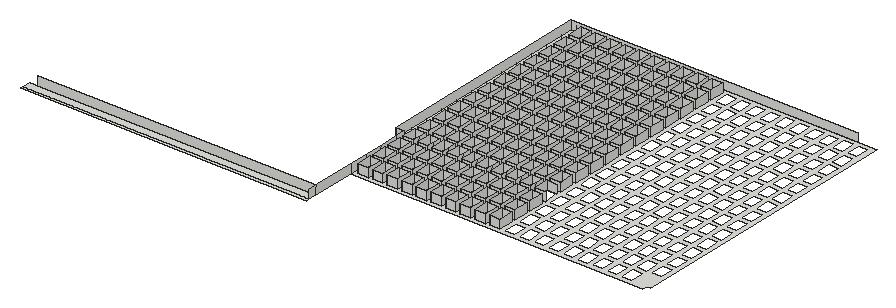
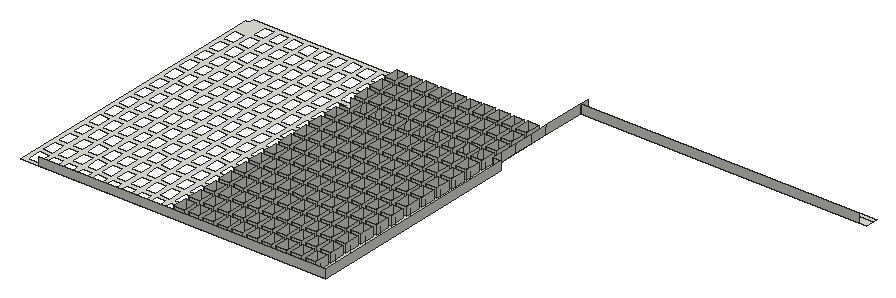
# SketchUp Ruby script. Lengths in inches.
U = 1.inch
M = Sketchup.active_model
def pt(a) = Geom::Point3d.new(a.map { |v| v * U })
def face(e, loops, mat)
  f = e.add_face(loops[0].map { |a| pt(a) })
  loops[1..].each { |l| e.add_face(l.map { |a| pt(a) }).erase! }
  f.material = f.back_material = mat if mat
  f
end
# faces: each face lists its corners as indices into pts; further lists are holes
def faces(e, pts, list, mat = nil) = list.each { |f| face(e, (f[0].is_a?(Array) ? f : [f]).map { |l| l.map { |i| pts[i] } }, mat) }
# xy, xz, yz: faces in a plane at the given z, y or x. An outline is a flat list of corners, or four numbers for a rectangle; further outlines are holes
def ring(l) = l.size == 4 ? [[l[0], l[1]], [l[2], l[1]], [l[2], l[3]], [l[0], l[3]]] : l.each_slice(2).to_a
def flat(e, list, mat, &to3) = list.each { |f| face(e, (f[0].is_a?(Array) ? f : [f]).map { |l| ring(l).map { |u, v| to3.(u, v) } }, mat) }
def xy(e, z, list, mat = nil) = flat(e, list, mat) { |x, y| [x, y, z] }
def xz(e, y, list, mat = nil) = flat(e, list, mat) { |x, z| [x, y, z] }
def yz(e, x, list, mat = nil) = flat(e, list, mat) { |y, z| [x, y, z] }
def lines(e, pts, list) = list.each { |a, b| e.add_line(pt(pts[a]), pt(pts[b])) }
# prism: a flat outline (further loops are holes) pulled along v
def prism(e, loops, v, mat = nil)
  f = face(e, loops, mat); d = Geom::Vector3d.new(v.map { |x| x * U })
  f.pushpull(f.normal.samedirection?(d) ? d.length : -d.length)
end
def box(e, o, s, mat = nil) = prism(e, [[o, [o[0] + s[0], o[1], o[2]], [o[0] + s[0], o[1] + s[1], o[2]], [o[0], o[1] + s[1], o[2]]]], [0, 0, s[2]], mat)
def at(x, y, z, deg = 0) = Geom::Transformation.translation(pt([x, y, z])) * Geom::Transformation.rotation(ORIGIN, Z_AXIS, deg.degrees)
def axes(o, x, y, z) = Geom::Transformation.new([*x, 0, *y, 0, *z, 0, *pt(o).to_a, 1])
def part(name) = M.definitions.add(name)
# library, detail: a bought-in or finely detailed component or shape, given as its bounding box
def library(name, o, s) = part(name).tap { |d| box(d.entities, o, s) }
def detail(e, o, s) = box(e.add_group.entities, o, s)
def put(e, d, t, mat = nil) = e.add_instance(d, t).tap { |i| i.material = mat if mat }
def group(e, t, mat = nil) = e.add_group.tap { |g| g.transformation = t; g.material = mat if mat }.entities
root = M.entities
xy(root,246,[[189.37,0.36,387.37,2.36],[189.37,2.36,387.37,8.36],[[387.37,38.27,387.37,84.36,381.37,84.36,381.37,236.18,592.3,236.18,592.3,41,589.58,41,589.58,38.27],[582.19,54.01,589.58,64.3],[582.19,93.05,589.58,103.33],[582.19,106.06,589.58,116.34],[582.19,223.16,589.58,233.45],[582.19,184.13,589.58,194.41],[582.19,145.09,589.58,155.38],[572.08,54.01,579.47,64.3],[572.08,93.05,579.47,103.33],[572.08,106.06,579.47,116.34],[572.08,145.09,579.47,155.38],[572.08,184.13,579.47,194.41],[572.08,223.16,579.47,233.45],[561.97,223.16,569.35,233.45],[561.97,184.13,569.35,194.41],[561.97,171.12,569.35,181.4],[561.97,145.09,569.35,155.38],[561.97,106.06,569.35,116.34],[561.97,93.05,569.35,103.33],[561.97,54.01,569.35,64.3],[390.09,223.16,397.48,233.45],[400.2,223.16,407.59,233.45],[400.2,184.13,407.59,194.41],[400.2,171.12,407.59,181.4],[400.2,145.09,407.59,155.38],[400.2,106.06,407.59,116.34],[400.2,93.05,407.59,103.33],[400.2,54.01,407.59,64.3],[410.3125,54.01,417.7,64.3],[410.3125,93.05,417.7,103.33],[410.3125,106.06,417.7,116.34],[410.3125,145.09,417.7,155.38],[410.3125,184.13,417.7,194.41],[410.3125,223.16,417.7,233.45],[420.42,223.16,427.81,233.45],[420.42,184.13,427.81,194.41],[420.42,145.09,427.81,155.38],[420.42,106.06,427.81,116.34],[420.42,93.05,427.81,103.33],[420.42,54.01,427.81,64.3],[430.53,223.16,437.92,233.45],[430.53,184.13,437.92,194.41],[430.53,145.09,437.92,155.38],[430.53,106.06,437.92,116.34],[430.53,93.05,437.92,103.33],[430.53,54.01,437.92,64.3],[440.64,54.01,448.03,64.3],[440.64,93.05,448.03,103.33],[440.64,106.06,448.03,116.34],[440.64,145.09,448.03,155.38],[440.64,184.13,448.03,194.41],[440.64,223.16,448.03,233.45],[450.75,223.16,458.14,233.45],[450.75,184.13,458.14,194.41],[450.75,145.09,458.14,155.38],[450.75,106.06,458.14,116.34],[450.75,93.05,458.14,103.33],[450.75,54.01,458.14,64.3],[470.97,54.01,478.36,64.3],[481.09,54.01,488.47,64.3],[491.2,54.01,498.58,64.3],[501.31,54.01,508.69,64.3],[511.42,54.01,518.8,64.3],[521.53,54.01,528.91,64.3],[531.64,54.01,539.02,64.3],[541.75,54.01,549.13,64.3],[551.86,54.01,559.24,64.3],[511.42,93.05,518.8,103.33],[511.42,106.06,518.8,116.34],[501.31,93.05,508.69,103.33],[491.2,93.05,498.58,103.33],[481.09,93.05,488.47,103.33],[470.97,93.05,478.36,103.33],[470.97,106.06,478.36,116.34],[481.09,106.06,488.47,116.34],[491.2,106.06,498.58,116.34],[501.31,106.06,508.69,116.34],[531.64,93.05,539.02,103.33],[541.75,93.05,549.13,103.33],[521.53,93.05,528.91,103.33],[551.86,93.05,559.24,103.33],[551.86,106.06,559.24,116.34],[541.75,106.06,549.13,116.34],[531.64,106.06,539.02,116.34],[521.53,106.06,528.91,116.34],[551.86,223.16,559.24,233.45],[551.86,184.13,559.24,194.41],[551.86,145.09,559.24,155.38],[541.75,145.09,549.13,155.38],[541.75,171.12,549.13,181.4],[541.75,184.13,549.13,194.41],[531.64,145.09,539.02,155.38],[541.75,223.16,549.13,233.45],[531.64,223.16,539.02,233.45],[531.64,184.13,539.02,194.41],[531.64,171.12,539.02,181.4],[521.53,184.13,528.91,194.41],[521.53,223.16,528.91,233.45],[521.53,145.09,528.91,155.38],[511.42,145.09,518.8,155.38],[511.42,171.12,518.8,181.4],[511.42,184.13,518.8,194.41],[511.42,223.16,518.8,233.45],[501.31,223.16,508.69,233.45],[501.31,184.13,508.69,194.41],[501.31,145.09,508.69,155.38],[470.97,145.09,478.36,155.38],[481.09,145.09,488.47,155.38],[491.2,145.09,498.58,155.38],[491.2,184.13,498.58,194.41],[481.09,184.13,488.47,194.41],[470.97,184.13,478.36,194.41],[470.97,223.16,478.36,233.45],[481.09,223.16,488.47,233.45],[491.2,223.16,498.58,233.45],[572.08,41,579.47,51.29],[410.3125,41,417.7,51.29],[440.64,41,448.03,51.29],[521.53,41,528.91,51.29],[491.2,41,498.58,51.29],[582.19,80.03,589.58,90.32],[572.08,80.03,579.47,90.32],[561.97,80.03,569.35,90.32],[400.2,80.03,407.59,90.32],[410.3125,80.03,417.7,90.32],[420.42,80.03,427.81,90.32],[430.53,80.03,437.92,90.32],[440.64,80.03,448.03,90.32],[450.75,80.03,458.14,90.32],[470.97,80.03,478.36,90.32],[481.09,80.03,488.47,90.32],[491.2,80.03,498.58,90.32],[501.31,80.03,508.69,90.32],[511.42,80.03,518.8,90.32],[521.53,80.03,528.91,90.32],[551.86,80.03,559.24,90.32],[541.75,80.03,549.13,90.32],[531.64,80.03,539.02,90.32],[582.19,67.02,589.58,77.31],[582.19,119.07,589.58,129.36],[582.19,132.08,589.58,142.37],[582.19,171.12,589.58,181.4],[582.19,158.1,589.58,168.39],[572.08,67.02,579.47,77.31],[572.08,119.07,579.47,129.36],[572.08,132.08,579.47,142.37],[572.08,158.1,579.47,168.39],[561.97,158.1,569.35,168.39],[561.97,132.08,569.35,142.37],[561.97,119.07,569.35,129.36],[561.97,67.02,569.35,77.31],[561.97,41,569.35,51.29],[400.2,158.1,407.59,168.39],[400.2,132.08,407.59,142.37],[400.2,119.07,407.59,129.36],[400.2,67.02,407.59,77.31],[400.2,41,407.59,51.29],[410.3125,67.02,417.7,77.31],[410.3125,119.07,417.7,129.36],[410.3125,132.08,417.7,142.37],[410.3125,158.1,417.7,168.39],[420.42,158.1,427.81,168.39],[420.42,132.08,427.81,142.37],[420.42,119.07,427.81,129.36],[420.42,67.02,427.81,77.31],[420.42,41,427.81,51.29],[430.53,171.12,437.92,181.4],[430.53,158.1,437.92,168.39],[430.53,132.08,437.92,142.37],[430.53,119.07,437.92,129.36],[430.53,67.02,437.92,77.31],[440.64,67.02,448.03,77.31],[440.64,119.07,448.03,129.36],[440.64,132.08,448.03,142.37],[440.64,158.1,448.03,168.39],[450.75,171.12,458.14,181.4],[450.75,158.1,458.14,168.39],[450.75,132.08,458.14,142.37],[450.75,119.07,458.14,129.36],[450.75,67.02,458.14,77.31],[450.75,41,458.14,51.29],[551.86,41,559.24,51.29],[531.64,41,539.02,51.29],[501.31,41,508.69,51.29],[481.09,41,488.47,51.29],[470.97,41,478.36,51.29],[470.97,67.02,478.36,77.31],[481.09,67.02,488.47,77.31],[491.2,67.02,498.58,77.31],[501.31,67.02,508.69,77.31],[511.42,67.02,518.8,77.31],[521.53,67.02,528.91,77.31],[531.64,67.02,539.02,77.31],[541.75,67.02,549.13,77.31],[551.86,67.02,559.24,77.31],[521.53,119.07,528.91,129.36],[531.64,119.07,539.02,129.36],[541.75,119.07,549.13,129.36],[551.86,119.07,559.24,129.36],[511.42,119.07,518.8,129.36],[501.31,119.07,508.69,129.36],[491.2,119.07,498.58,129.36],[481.09,119.07,488.47,129.36],[470.97,119.07,478.36,129.36],[551.86,158.1,559.24,168.39],[551.86,132.08,559.24,142.37],[541.75,158.1,549.13,168.39],[541.75,132.08,549.13,142.37],[531.64,132.08,539.02,142.37],[531.64,158.1,539.02,168.39],[521.53,171.12,528.91,181.4],[521.53,158.1,528.91,168.39],[521.53,132.08,528.91,142.37],[511.42,132.08,518.8,142.37],[511.42,158.1,518.8,168.39],[501.31,171.12,508.69,181.4],[501.31,158.1,508.69,168.39],[501.31,132.08,508.69,142.37],[481.09,132.08,488.47,142.37],[470.97,132.08,478.36,142.37],[491.2,132.08,498.58,142.37],[491.2,158.1,498.58,168.39],[481.09,158.1,488.47,168.39],[470.97,158.1,478.36,168.39],[470.97,171.12,478.36,181.4],[481.09,171.12,488.47,181.4],[491.2,171.12,498.58,181.4],[430.53,41,437.92,51.29],[541.75,41,549.13,51.29],[511.42,41,518.8,51.29],[582.19,210.15,589.58,220.4375],[582.19,197.14,589.58,207.43],[572.08,171.12,579.47,181.4],[572.08,197.14,579.47,207.43],[572.08,210.15,579.47,220.4375],[561.97,210.15,569.35,220.4375],[561.97,197.14,569.35,207.43],[400.2,210.15,407.59,220.4375],[400.2,197.14,407.59,207.43],[410.3125,171.12,417.7,181.4],[410.3125,197.14,417.7,207.43],[410.3125,210.15,417.7,220.4375],[420.42,210.15,427.81,220.4375],[420.42,197.14,427.81,207.43],[420.42,171.12,427.81,181.4],[430.53,210.15,437.92,220.4375],[430.53,197.14,437.92,207.43],[440.64,171.12,448.03,181.4],[440.64,197.14,448.03,207.43],[440.64,210.15,448.03,220.4375],[450.75,210.15,458.14,220.4375],[450.75,197.14,458.14,207.43],[551.86,210.15,559.24,220.4375],[551.86,197.14,559.24,207.43],[551.86,171.12,559.24,181.4],[541.75,197.14,549.13,207.43],[541.75,210.15,549.13,220.4375],[531.64,210.15,539.02,220.4375],[531.64,197.14,539.02,207.43],[521.53,197.14,528.91,207.43],[521.53,210.15,528.91,220.4375],[511.42,197.14,518.8,207.43],[511.42,210.15,518.8,220.4375],[501.31,210.15,508.69,220.4375],[501.31,197.14,508.69,207.43],[470.97,197.14,478.36,207.43],[481.09,197.14,488.47,207.43],[491.2,197.14,498.58,207.43],[491.2,210.15,498.58,220.4375],[481.09,210.15,488.47,220.4375],[470.97,210.15,478.36,220.4375],[390.09,54.01,397.48,64.3],[390.09,93.05,397.48,103.33],[390.09,106.06,397.48,116.34],[390.09,145.09,397.48,155.38],[390.09,184.13,397.48,194.41],[390.09,41,397.48,51.29],[390.09,67.02,397.48,77.31],[390.09,80.03,397.48,90.32],[390.09,119.07,397.48,129.36],[390.09,132.08,397.48,142.37],[390.09,158.1,397.48,168.39],[390.09,171.12,397.48,181.4],[390.09,197.14,397.48,207.43],[390.09,210.15,397.48,220.4375],[460.86,223.16,468.25,233.45],[460.86,184.13,468.25,194.41],[460.86,145.09,468.25,155.38],[460.86,106.06,468.25,116.34],[460.86,93.05,468.25,103.33],[460.86,54.01,468.25,64.3],[460.86,171.12,468.25,181.4],[460.86,158.1,468.25,168.39],[460.86,132.08,468.25,142.37],[460.86,119.07,468.25,129.36],[460.86,80.03,468.25,90.32],[460.86,67.02,468.25,77.31],[460.86,41,468.25,51.29],[460.86,210.15,468.25,220.4375],[460.86,197.14,468.25,207.43]]])
xz(root,8.36,[[195.37,246,387.37,252]])
xz(root,41,[[390.09,246,397.48,252],[400.2,246,407.59,252],[410.3125,246,417.7,252],[420.42,246,427.81,252],[430.53,246,437.92,252],
  [440.64,246,448.03,252],[450.75,246,458.14,252],[460.86,246,468.25,252],[470.97,246,478.36,252],[481.09,246,488.47,252]])
xz(root,51.29,[[390.09,246,397.48,252],[400.2,246,407.59,252],[410.3125,246,417.7,252],[420.42,246,427.81,252],[430.53,246,437.92,252],
  [440.64,246,448.03,252],[450.75,246,458.14,252],[460.86,246,468.25,252],[470.97,246,478.36,252],[481.09,246,488.47,252]])
xz(root,54.01,[[390.09,246,397.48,252],[400.2,246,407.59,252],[410.3125,246,417.7,252],[420.42,246,427.81,252],[430.53,246,437.92,252],
  [440.64,246,448.03,252],[450.75,246,458.14,252],[460.86,246,468.25,252],[470.97,246,478.36,252],[481.09,246,488.47,252]])
xz(root,64.3,[[390.09,246,397.48,252],[400.2,246,407.59,252],[410.3125,246,417.7,252],[420.42,246,427.81,252],[430.53,246,437.92,252],
  [440.64,246,448.03,252],[450.75,246,458.14,252],[460.86,246,468.25,252],[470.97,246,478.36,252],[481.09,246,488.47,252]])
xz(root,67.02,[[390.09,246,397.48,252],[400.2,246,407.59,252],[410.3125,246,417.7,252],[420.42,246,427.81,252],[430.53,246,437.92,252],
  [440.64,246,448.03,252],[450.75,246,458.14,252],[460.86,246,468.25,252],[470.97,246,478.36,252],[481.09,246,488.47,252]])
xz(root,77.31,[[390.09,246,397.48,252],[400.2,246,407.59,252],[410.3125,246,417.7,252],[420.42,246,427.81,252],[430.53,246,437.92,252],
  [440.64,246,448.03,252],[450.75,246,458.14,252],[460.86,246,468.25,252],[470.97,246,478.36,252],[481.09,246,488.47,252]])
xz(root,80.03,[[390.09,246,397.48,252],[400.2,246,407.59,252],[410.3125,246,417.7,252],[420.42,246,427.81,252],[430.53,246,437.92,252],
  [440.64,246,448.03,252],[450.75,246,458.14,252],[460.86,246,468.25,252],[470.97,246,478.36,252],[481.09,246,488.47,252]])
xz(root,84.36,[[381.37,246,387.37,252]])
xz(root,90.32,[[390.09,246,397.48,252],[400.2,246,407.59,252],[410.3125,246,417.7,252],[420.42,246,427.81,252],[430.53,246,437.92,252],
  [440.64,246,448.03,252],[450.75,246,458.14,252],[460.86,246,468.25,252],[470.97,246,478.36,252],[481.09,246,488.47,252]])
xz(root,93.05,[[390.09,246,397.48,252],[400.2,246,407.59,252],[410.3125,246,417.7,252],[420.42,246,427.81,252],[430.53,246,437.92,252],
  [440.64,246,448.03,252],[450.75,246,458.14,252],[460.86,246,468.25,252],[470.97,246,478.36,252],[481.09,246,488.47,252]])
xz(root,103.33,[[390.09,246,397.48,252],[400.2,246,407.59,252],[410.3125,246,417.7,252],[420.42,246,427.81,252],[430.53,246,437.92,252],
  [440.64,246,448.03,252],[450.75,246,458.14,252],[460.86,246,468.25,252],[470.97,246,478.36,252],[481.09,246,488.47,252]])
xz(root,106.06,[[390.09,246,397.48,252],[400.2,246,407.59,252],[410.3125,246,417.7,252],[420.42,246,427.81,252],[430.53,246,437.92,252],
  [440.64,246,448.03,252],[450.75,246,458.14,252],[460.86,246,468.25,252],[470.97,246,478.36,252],[481.09,246,488.47,252]])
xz(root,116.34,[[390.09,246,397.48,252],[400.2,246,407.59,252],[410.3125,246,417.7,252],[420.42,246,427.81,252],[430.53,246,437.92,252],
  [440.64,246,448.03,252],[450.75,246,458.14,252],[460.86,246,468.25,252],[470.97,246,478.36,252],[481.09,246,488.47,252]])
xz(root,119.07,[[390.09,246,397.48,252],[400.2,246,407.59,252],[410.3125,246,417.7,252],[420.42,246,427.81,252],[430.53,246,437.92,252],
  [440.64,246,448.03,252],[450.75,246,458.14,252],[460.86,246,468.25,252],[470.97,246,478.36,252],[481.09,246,488.47,252]])
xz(root,129.36,[[390.09,246,397.48,252],[400.2,246,407.59,252],[410.3125,246,417.7,252],[420.42,246,427.81,252],[430.53,246,437.92,252],
  [440.64,246,448.03,252],[450.75,246,458.14,252],[460.86,246,468.25,252],[470.97,246,478.36,252],[481.09,246,488.47,252]])
xz(root,132.08,[[390.09,246,397.48,252],[400.2,246,407.59,252],[410.3125,246,417.7,252],[420.42,246,427.81,252],[430.53,246,437.92,252],
  [440.64,246,448.03,252],[450.75,246,458.14,252],[460.86,246,468.25,252],[470.97,246,478.36,252],[481.09,246,488.47,252]])
xz(root,142.37,[[390.09,246,397.48,252],[400.2,246,407.59,252],[410.3125,246,417.7,252],[420.42,246,427.81,252],[430.53,246,437.92,252],
  [440.64,246,448.03,252],[450.75,246,458.14,252],[460.86,246,468.25,252],[470.97,246,478.36,252],[481.09,246,488.47,252]])
xz(root,145.09,[[390.09,246,397.48,252],[400.2,246,407.59,252],[410.3125,246,417.7,252],[420.42,246,427.81,252],[430.53,246,437.92,252],
  [440.64,246,448.03,252],[450.75,246,458.14,252],[460.86,246,468.25,252],[470.97,246,478.36,252],[481.09,246,488.47,252]])
xz(root,155.38,[[390.09,246,397.48,252],[400.2,246,407.59,252],[410.3125,246,417.7,252],[420.42,246,427.81,252],[430.53,246,437.92,252],
  [440.64,246,448.03,252],[450.75,246,458.14,252],[460.86,246,468.25,252],[470.97,246,478.36,252],[481.09,246,488.47,252]])
xz(root,158.1,[[390.09,246,397.48,252],[400.2,246,407.59,252],[410.3125,246,417.7,252],[420.42,246,427.81,252],[430.53,246,437.92,252],
  [440.64,246,448.03,252],[450.75,246,458.14,252],[460.86,246,468.25,252],[470.97,246,478.36,252],[481.09,246,488.47,252]])
xz(root,168.39,[[390.09,246,397.48,252],[400.2,246,407.59,252],[410.3125,246,417.7,252],[420.42,246,427.81,252],[430.53,246,437.92,252],
  [440.64,246,448.03,252],[450.75,246,458.14,252],[460.86,246,468.25,252],[470.97,246,478.36,252],[481.09,246,488.47,252]])
xz(root,171.12,[[390.09,246,397.48,252],[400.2,246,407.59,252],[410.3125,246,417.7,252],[420.42,246,427.81,252],[430.53,246,437.92,252],
  [440.64,246,448.03,252],[450.75,246,458.14,252],[460.86,246,468.25,252],[470.97,246,478.36,252],[481.09,246,488.47,252]])
xz(root,181.4,[[390.09,246,397.48,252],[400.2,246,407.59,252],[410.3125,246,417.7,252],[420.42,246,427.81,252],[430.53,246,437.92,252],
  [440.64,246,448.03,252],[450.75,246,458.14,252],[460.86,246,468.25,252],[470.97,246,478.36,252],[481.09,246,488.47,252]])
xz(root,184.13,[[390.09,246,397.48,252],[400.2,246,407.59,252],[410.3125,246,417.7,252],[420.42,246,427.81,252],[430.53,246,437.92,252],
  [440.64,246,448.03,252],[450.75,246,458.14,252],[460.86,246,468.25,252],[470.97,246,478.36,252],[481.09,246,488.47,252]])
xz(root,194.41,[[390.09,246,397.48,252],[400.2,246,407.59,252],[410.3125,246,417.7,252],[420.42,246,427.81,252],[430.53,246,437.92,252],
  [440.64,246,448.03,252],[450.75,246,458.14,252],[460.86,246,468.25,252],[470.97,246,478.36,252],[481.09,246,488.47,252]])
xz(root,197.14,[[390.09,246,397.48,252],[400.2,246,407.59,252],[410.3125,246,417.7,252],[420.42,246,427.81,252],[430.53,246,437.92,252],
  [440.64,246,448.03,252],[450.75,246,458.14,252],[460.86,246,468.25,252],[470.97,246,478.36,252],[481.09,246,488.47,252]])
xz(root,207.43,[[390.09,246,397.48,252],[400.2,246,407.59,252],[410.3125,246,417.7,252],[420.42,246,427.81,252],[430.53,246,437.92,252],
  [440.64,246,448.03,252],[450.75,246,458.14,252],[460.86,246,468.25,252],[470.97,246,478.36,252],[481.09,246,488.47,252]])
xz(root,210.15,[[390.09,246,397.48,252],[400.2,246,407.59,252],[410.3125,246,417.7,252],[420.42,246,427.81,252],[430.53,246,437.92,252],
  [440.64,246,448.03,252],[450.75,246,458.14,252],[460.86,246,468.25,252],[470.97,246,478.36,252],[481.09,246,488.47,252]])
xz(root,220.4375,[[390.09,246,397.48,252],[400.2,246,407.59,252],[410.3125,246,417.7,252],[420.42,246,427.81,252],[430.53,246,437.92,252],
  [440.64,246,448.03,252],[450.75,246,458.14,252],[460.86,246,468.25,252],[470.97,246,478.36,252],[481.09,246,488.47,252]])
xz(root,223.16,[[390.09,246,397.48,252],[400.2,246,407.59,252],[410.3125,246,417.7,252],[420.42,246,427.81,252],[430.53,246,437.92,252],
  [440.64,246,448.03,252],[450.75,246,458.14,252],[460.86,246,468.25,252],[470.97,246,478.36,252],[481.09,246,488.47,252]])
xz(root,233.45,[[390.09,246,397.48,252],[400.2,246,407.59,252],[410.3125,246,417.7,252],[420.42,246,427.81,252],[430.53,246,437.92,252],
  [440.64,246,448.03,252],[450.75,246,458.14,252],[460.86,246,468.25,252],[470.97,246,478.36,252],[481.09,246,488.47,252]])
xz(root,236.18,[[381.37,246,579.37,252]])
yz(root,381.37,[[84.36,246,236.18,252]])
yz(root,387.37,[[2.36,246,8.36,252],[8.36,246,38.27,252],[38.27,246,51.29,252],[51.29,246,64.3,252],[64.3,246,77.31,252],
  [77.31,246,84.36,252]])
yz(root,390.09,[[41,246,51.29,252],[54.01,246,64.3,252],[67.02,246,77.31,252],[80.03,246,90.32,252],[93.05,246,103.33,252],
  [106.06,246,116.34,252],[119.07,246,129.36,252],[132.08,246,142.37,252],[145.09,246,155.38,252],[158.1,246,168.39,252],
  [171.12,246,181.4,252],[184.13,246,194.41,252],[197.14,246,207.43,252],[210.15,246,220.4375,252],[223.16,246,233.45,252]])
yz(root,397.48,[[41,246,51.29,252],[54.01,246,64.3,252],[67.02,246,77.31,252],[80.03,246,84.36,252],[84.36,246,90.32,252],
  [93.05,246,103.33,252],[106.06,246,116.34,252],[119.07,246,129.36,252],[132.08,246,142.37,252],[145.09,246,155.38,252],
  [158.1,246,168.39,252],[171.12,246,181.4,252],[184.13,246,194.41,252],[197.14,246,207.43,252],[210.15,246,220.4375,252],
  [223.16,246,233.45,252]])
yz(root,400.2,[[41,246,51.29,252],[54.01,246,64.3,252],[67.02,246,77.31,252],[80.03,246,90.32,252],[93.05,246,103.33,252],
  [106.06,246,116.34,252],[119.07,246,129.36,252],[132.08,246,142.37,252],[145.09,246,155.38,252],[158.1,246,168.39,252],
  [171.12,246,181.4,252],[184.13,246,194.41,252],[197.14,246,207.43,252],[210.15,246,220.4375,252],[223.16,246,233.45,252]])
yz(root,407.59,[[41,246,51.29,252],[54.01,246,64.3,252],[67.02,246,77.31,252],[80.03,246,84.36,252],[84.36,246,90.32,252],
  [93.05,246,103.33,252],[106.06,246,116.34,252],[119.07,246,129.36,252],[132.08,246,142.37,252],[145.09,246,155.38,252],
  [158.1,246,168.39,252],[171.12,246,181.4,252],[184.13,246,194.41,252],[197.14,246,207.43,252],[210.15,246,220.4375,252],
  [223.16,246,233.45,252]])
yz(root,410.3125,[[41,246,51.29,252],[54.01,246,64.3,252],[67.02,246,77.31,252],[80.03,246,90.32,252],[93.05,246,103.33,252],
  [106.06,246,116.34,252],[119.07,246,129.36,252],[132.08,246,142.37,252],[145.09,246,155.38,252],[158.1,246,168.39,252],
  [171.12,246,181.4,252],[184.13,246,194.41,252],[197.14,246,207.43,252],[210.15,246,220.4375,252],[223.16,246,233.45,252]])
yz(root,417.7,[[41,246,51.29,252],[54.01,246,64.3,252],[67.02,246,77.31,252],[80.03,246,84.36,252],[84.36,246,90.32,252],
  [93.05,246,103.33,252],[106.06,246,116.34,252],[119.07,246,129.36,252],[132.08,246,142.37,252],[145.09,246,155.38,252],
  [158.1,246,168.39,252],[171.12,246,181.4,252],[184.13,246,194.41,252],[197.14,246,207.43,252],[210.15,246,220.4375,252],
  [223.16,246,233.45,252]])
yz(root,420.42,[[41,246,51.29,252],[54.01,246,64.3,252],[67.02,246,77.31,252],[80.03,246,90.32,252],[93.05,246,103.33,252],
  [106.06,246,116.34,252],[119.07,246,129.36,252],[132.08,246,142.37,252],[145.09,246,155.38,252],[158.1,246,168.39,252],
  [171.12,246,181.4,252],[184.13,246,194.41,252],[197.14,246,207.43,252],[210.15,246,220.4375,252],[223.16,246,233.45,252]])
yz(root,427.81,[[41,246,51.29,252],[54.01,246,64.3,252],[67.02,246,77.31,252],[80.03,246,84.36,252],[84.36,246,90.32,252],
  [93.05,246,103.33,252],[106.06,246,116.34,252],[119.07,246,129.36,252],[132.08,246,142.37,252],[145.09,246,155.38,252],
  [158.1,246,168.39,252],[171.12,246,181.4,252],[184.13,246,194.41,252],[197.14,246,207.43,252],[210.15,246,220.4375,252],
  [223.16,246,233.45,252]])
yz(root,430.53,[[41,246,51.29,252],[54.01,246,64.3,252],[67.02,246,77.31,252],[80.03,246,90.32,252],[93.05,246,103.33,252],
  [106.06,246,116.34,252],[119.07,246,129.36,252],[132.08,246,142.37,252],[145.09,246,155.38,252],[158.1,246,168.39,252],
  [171.12,246,181.4,252],[184.13,246,194.41,252],[197.14,246,207.43,252],[210.15,246,220.4375,252],[223.16,246,233.45,252]])
yz(root,437.92,[[41,246,51.29,252],[54.01,246,64.3,252],[67.02,246,77.31,252],[80.03,246,84.36,252],[84.36,246,90.32,252],
  [93.05,246,103.33,252],[106.06,246,116.34,252],[119.07,246,129.36,252],[132.08,246,142.37,252],[145.09,246,155.38,252],
  [158.1,246,168.39,252],[171.12,246,181.4,252],[184.13,246,194.41,252],[197.14,246,207.43,252],[210.15,246,220.4375,252],
  [223.16,246,233.45,252]])
yz(root,440.64,[[41,246,51.29,252],[54.01,246,64.3,252],[67.02,246,77.31,252],[80.03,246,90.32,252],[93.05,246,103.33,252],
  [106.06,246,116.34,252],[119.07,246,129.36,252],[132.08,246,142.37,252],[145.09,246,155.38,252],[158.1,246,168.39,252],
  [171.12,246,181.4,252],[184.13,246,194.41,252],[197.14,246,207.43,252],[210.15,246,220.4375,252],[223.16,246,233.45,252]])
yz(root,448.03,[[41,246,51.29,252],[54.01,246,64.3,252],[67.02,246,77.31,252],[80.03,246,84.36,252],[84.36,246,90.32,252],
  [93.05,246,103.33,252],[106.06,246,116.34,252],[119.07,246,129.36,252],[132.08,246,142.37,252],[145.09,246,155.38,252],
  [158.1,246,168.39,252],[171.12,246,181.4,252],[184.13,246,194.41,252],[197.14,246,207.43,252],[210.15,246,220.4375,252],
  [223.16,246,233.45,252]])
yz(root,450.75,[[41,246,51.29,252],[54.01,246,64.3,252],[67.02,246,77.31,252],[80.03,246,90.32,252],[93.05,246,103.33,252],
  [106.06,246,116.34,252],[119.07,246,129.36,252],[132.08,246,142.37,252],[145.09,246,155.38,252],[158.1,246,168.39,252],
  [171.12,246,181.4,252],[184.13,246,194.41,252],[197.14,246,207.43,252],[210.15,246,220.4375,252],[223.16,246,233.45,252]])
yz(root,458.14,[[41,246,51.29,252],[54.01,246,64.3,252],[67.02,246,77.31,252],[80.03,246,84.36,252],[84.36,246,90.32,252],
  [93.05,246,103.33,252],[106.06,246,116.34,252],[119.07,246,129.36,252],[132.08,246,142.37,252],[145.09,246,155.38,252],
  [158.1,246,168.39,252],[171.12,246,181.4,252],[184.13,246,194.41,252],[197.14,246,207.43,252],[210.15,246,220.4375,252],
  [223.16,246,233.45,252]])
yz(root,460.86,[[41,246,51.29,252],[54.01,246,64.3,252],[67.02,246,77.31,252],[80.03,246,90.32,252],[93.05,246,103.33,252],
  [106.06,246,116.34,252],[119.07,246,129.36,252],[132.08,246,142.37,252],[145.09,246,155.38,252],[158.1,246,168.39,252],
  [171.12,246,181.4,252],[184.13,246,194.41,252],[197.14,246,207.43,252],[210.15,246,220.4375,252],[223.16,246,233.45,252]])
yz(root,468.25,[[41,246,51.29,252],[54.01,246,64.3,252],[67.02,246,77.31,252],[80.03,246,84.36,252],[84.36,246,90.32,252],
  [93.05,246,103.33,252],[106.06,246,116.34,252],[119.07,246,129.36,252],[132.08,246,142.37,252],[145.09,246,155.38,252],
  [158.1,246,168.39,252],[171.12,246,181.4,252],[184.13,246,194.41,252],[197.14,246,207.43,252],[210.15,246,220.4375,252],
  [223.16,246,233.45,252]])
yz(root,470.97,[[41,246,51.29,252],[54.01,246,64.3,252],[67.02,246,77.31,252],[80.03,246,90.32,252],[93.05,246,103.33,252],
  [106.06,246,116.34,252],[119.07,246,129.36,252],[132.08,246,142.37,252],[145.09,246,155.38,252],[158.1,246,168.39,252],
  [171.12,246,181.4,252],[184.13,246,194.41,252],[197.14,246,207.43,252],[210.15,246,220.4375,252],[223.16,246,233.45,252]])
yz(root,478.36,[[41,246,51.29,252],[54.01,246,64.3,252],[67.02,246,77.31,252],[80.03,246,84.36,252],[84.36,246,90.32,252],
  [93.05,246,103.33,252],[106.06,246,116.34,252],[119.07,246,129.36,252],[132.08,246,142.37,252],[145.09,246,155.38,252],
  [158.1,246,168.39,252],[171.12,246,181.4,252],[184.13,246,194.41,252],[197.14,246,207.43,252],[210.15,246,220.4375,252],
  [223.16,246,233.45,252]])
yz(root,481.09,[[41,246,51.29,252],[54.01,246,64.3,252],[67.02,246,77.31,252],[80.03,246,90.32,252],[93.05,246,103.33,252],
  [106.06,246,116.34,252],[119.07,246,129.36,252],[132.08,246,142.37,252],[145.09,246,155.38,252],[158.1,246,168.39,252],
  [171.12,246,181.4,252],[184.13,246,194.41,252],[197.14,246,207.43,252],[210.15,246,220.4375,252],[223.16,246,233.45,252]])
yz(root,488.47,[[41,246,51.29,252],[54.01,246,64.3,252],[67.02,246,77.31,252],[93.05,246,103.33,252],[106.06,246,116.34,252],
  [119.07,246,129.36,252],[132.08,246,142.37,252],[145.09,246,155.38,252],[158.1,246,168.39,252],[171.12,246,181.4,252],
  [184.13,246,194.41,252],[197.14,246,207.43,252],[210.15,246,220.4375,252],[223.16,246,233.45,252]])
p = [[387.37,90.32,252],[387.37,90.32,246],[387.37,103.33,252],[387.37,103.33,246],[387.37,116.34,252],[387.37,116.34,246],
  [387.37,129.36,252],[387.37,129.36,246],[387.37,142.37,252],[387.37,142.37,246],[387.37,155.38,252],[387.37,155.38,246],
  [387.37,168.39,252],[387.37,168.39,246],[387.37,181.4,252],[387.37,181.4,246],[387.37,194.41,252],[387.37,194.41,246],
  [387.37,207.43,252],[387.37,207.43,246],[387.37,220.4375,252],[387.37,220.4375,246],[387.37,233.45,252],[387.37,233.45,246]]
lines(root,p,[[0,1],[2,3],[4,5],[6,7],[8,9],[10,11],[12,13],[14,15],[16,17],[18,19],[20,21],[22,23]])
